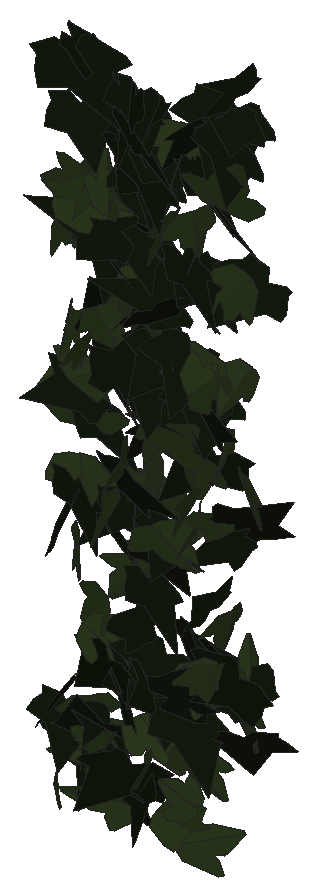
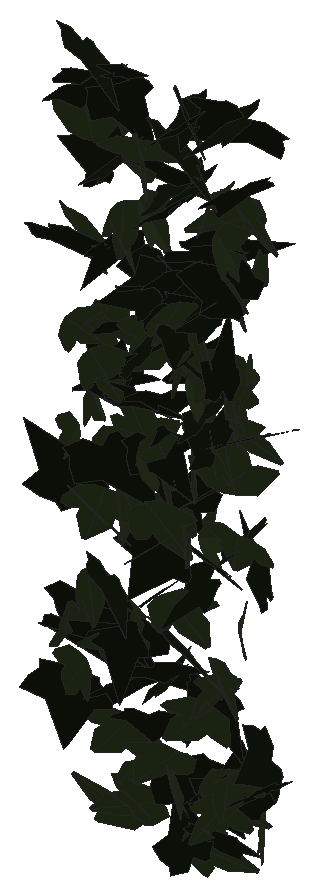
# SketchUp Ruby script. Lengths in inches.
U = 1.inch
M = Sketchup.active_model
def pt(a) = Geom::Point3d.new(a.map { |v| v * U })
def face(e, loops, mat)
  f = e.add_face(loops[0].map { |a| pt(a) })
  loops[1..].each { |l| e.add_face(l.map { |a| pt(a) }).erase! }
  f.material = f.back_material = mat if mat
  f
end
# faces: each face lists its corners as indices into pts; further lists are holes
def faces(e, pts, list, mat = nil) = list.each { |f| face(e, (f[0].is_a?(Array) ? f : [f]).map { |l| l.map { |i| pts[i] } }, mat) }
# xy, xz, yz: faces in a plane at the given z, y or x. An outline is a flat list of corners, or four numbers for a rectangle; further outlines are holes
def ring(l) = l.size == 4 ? [[l[0], l[1]], [l[2], l[1]], [l[2], l[3]], [l[0], l[3]]] : l.each_slice(2).to_a
def flat(e, list, mat, &to3) = list.each { |f| face(e, (f[0].is_a?(Array) ? f : [f]).map { |l| ring(l).map { |u, v| to3.(u, v) } }, mat) }
def xy(e, z, list, mat = nil) = flat(e, list, mat) { |x, y| [x, y, z] }
def xz(e, y, list, mat = nil) = flat(e, list, mat) { |x, z| [x, y, z] }
def yz(e, x, list, mat = nil) = flat(e, list, mat) { |y, z| [x, y, z] }
def lines(e, pts, list) = list.each { |a, b| e.add_line(pt(pts[a]), pt(pts[b])) }
# prism: a flat outline (further loops are holes) pulled along v
def prism(e, loops, v, mat = nil)
  f = face(e, loops, mat); d = Geom::Vector3d.new(v.map { |x| x * U })
  f.pushpull(f.normal.samedirection?(d) ? d.length : -d.length)
end
def box(e, o, s, mat = nil) = prism(e, [[o, [o[0] + s[0], o[1], o[2]], [o[0] + s[0], o[1] + s[1], o[2]], [o[0], o[1] + s[1], o[2]]]], [0, 0, s[2]], mat)
def at(x, y, z, deg = 0) = Geom::Transformation.translation(pt([x, y, z])) * Geom::Transformation.rotation(ORIGIN, Z_AXIS, deg.degrees)
def axes(o, x, y, z) = Geom::Transformation.new([*x, 0, *y, 0, *z, 0, *pt(o).to_a, 1])
def part(name) = M.definitions.add(name)
# library, detail: a bought-in or finely detailed component or shape, given as its bounding box
def library(name, o, s) = part(name).tap { |d| box(d.entities, o, s) }
def detail(e, o, s) = box(e.add_group.entities, o, s)
def put(e, d, t, mat = nil) = e.add_instance(d, t).tap { |i| i.material = mat if mat }
def group(e, t, mat = nil) = e.add_group.tap { |g| g.transformation = t; g.material = mat if mat }.entities
root = M.entities
M.materials.add("1026 AP 7946 SUNNY SIDE UP").color = [254, 231, 186]
M.materials.add("efeu1").color = [18, 25, 13]
M.materials.add("efeu2").color = [43, 57, 29]
c1 = part("ivyleaf_10")
p = [[0,0.5,-0.03],[-0.0625,2.02,-0.43],[-0.19,2.01,-0.46],[-0.54,1.05,-0.29],[-0.52,0.625,-0.18],[-0.83,0.76,-0.28],
  [-1.16,0.64,-0.33],[-1.15,0.33,-0.24],[-0.77,-0.39,0.02],[-0.3,-0.51,0.16],[0.04,-0.48,0.23],[-0.02,2.01,-0.4375],
  [-0.06,2.01,-0.43],[0.04,-0.49,0.23],[0.67,-0.49,0.14],[1.38,0.36,-0.2],[1.375,0.51,-0.24],[0.81,0.65,-0.19],
  [0.62,0.59,-0.15],[0.6,1.09,-0.28],[0.5,1.23,-0.31]]
faces(c1.entities,p,[[0,1,2,3,4,5,6,7,8,9,10],[11,12,0,13,14,15,16,17,18,19,20]],"efeu2")
c2 = part("ivyleaf_9")
p = [[1.54,2.16,1.25],[1.36,2.04,1.19],[-0.21,0.99,0.68],[-0.71,1.11,0.82],[-0.85,0.86,0.67],[-0.8,0.17,0.21],
  [-0.9,-0.01,0.1],[-0.67,-0.16,-0.02],[-0.08,-0.08,-0.05],[-0.03,-0.6,-0.4],[0.65,-0.88,-0.66],[0.83,-0.6,-0.49],
  [1.29,-0.42,-0.43],[1.8125,-0.07,-0.26],[1.21,0.44,0.15]]
faces(c2.entities,p,[[0,1,2,3,4,5,6,7,8,9,10,11,12,13,14]],"efeu1")
put(root,c1,axes([121.98,211.52,277.31],[0.03171,0.08334,0.32849],[0.20526,0.2908,-0.08524],[-0.47506,0.13121,-0.0149]),"1026 AP 7946 SUNNY SIDE UP")
put(root,c2,axes([121.49,211.78,272],[0.02452,0.24373,0.23934],[-0.06911,-0.22772,0.24931],[0.52342,-0.04148,0.02171]),"1026 AP 7946 SUNNY SIDE UP")
put(root,c2,axes([122.73,211.57,274.8125],[-0.20002,-0.06797,0.29588],[0.33643,0.19479,0.14606],[-0.32051,0.24688,-0.03133]),"1026 AP 7946 SUNNY SIDE UP")
put(root,c1,axes([122,211.64,277.5],[0.1599,-0.14005,-0.28907],[-0.3313,0.18686,-0.17415],[0.36373,0.23176,-0.03154]),"1026 AP 7946 SUNNY SIDE UP")
put(root,c2,axes([123.08,212.01,270.04],[-0.16156,-0.09203,0.26941],[-0.07925,-0.26858,-0.1191],[0.42945,-0.08418,0.07937]),"1026 AP 7946 SUNNY SIDE UP")
put(root,c2,axes([123.3,211.59,276.1],[0.17775,0.27835,0.04444],[0.04748,0.03253,-0.30889],[-0.43998,0.11597,-0.01538]),"1026 AP 7946 SUNNY SIDE UP")
put(root,c1,axes([122.26,212,272.6],[0.0991,-0.11712,0.28965],[0.16515,-0.26187,-0.13784],[0.45057,0.12174,-0.01318]),"1026 AP 7946 SUNNY SIDE UP")
put(root,c2,axes([122.66,211.8,278.65],[0.36741,-0.24284,-0.07309],[-0.09666,0.03725,-0.34646],[0.38526,0.24093,-0.01722]),"1026 AP 7946 SUNNY SIDE UP")
put(root,c1,axes([124.17,211.77,270.86],[-0.29442,-0.23757,-0.04002],[0.06154,0.0168,-0.31083],[0.37314,-0.19022,0.01968]),"1026 AP 7946 SUNNY SIDE UP")
put(root,c2,axes([124.53,211.8,270.88],[0.10748,0.01102,-0.34467],[-0.45516,-0.16967,-0.06767],[-0.26453,0.29641,-0.02361]),"1026 AP 7946 SUNNY SIDE UP")
put(root,c1,axes([122.68,211.65,273.58],[0.01249,-0.2277,-0.23311],[-0.01185,0.22486,-0.2334],[0.50319,0.01094,0.00029]),"1026 AP 7946 SUNNY SIDE UP")
put(root,c2,axes([122.7,211.86,268.9],[0.12076,0.13717,-0.30129],[-0.16617,-0.27424,-0.16228],[-0.48116,0.12914,-0.01957]),"1026 AP 7946 SUNNY SIDE UP")
put(root,c2,axes([123.58,211.89,276.83],[0.15184,-0.28554,-0.01731],[-0.01676,0.01242,-0.31039],[0.44931,0.09696,-0.00573]),"1026 AP 7946 SUNNY SIDE UP")
put(root,c1,axes([123.93,211.76,270.77],[-0.28756,-0.03559,-0.23541],[0.35968,0.01327,-0.19081],[0.05136,-0.29222,0.01827]),"1026 AP 7946 SUNNY SIDE UP")
put(root,c1,axes([124.01,211.5625,275.1875],[0.09265,0.02287,-0.32986],[0.16457,0.30652,0.04417],[0.47738,-0.1101,0.04879]),"1026 AP 7946 SUNNY SIDE UP")
put(root,c2,axes([122.39,211.97,276.82],[-0.26474,-0.19951,-0.20035],[-0.10805,-0.18914,0.26162],[-0.42328,0.17307,0.05853]),"1026 AP 7946 SUNNY SIDE UP")
put(root,c2,axes([123.64,211.95,269.94],[-0.06302,-0.3296,-0.06102],[0.04817,0.05391,-0.34088],[0.52385,-0.04461,0.02401]),"1026 AP 7946 SUNNY SIDE UP")
put(root,c2,axes([123.62,212.01,275.38],[-0.23731,-0.27407,0.02875],[-0.00163,-0.03303,-0.32215],[0.43343,-0.15018,0.01453]),"1026 AP 7946 SUNNY SIDE UP")
put(root,c1,axes([124.33,211.84,277.98],[-0.50833,-0.04495,0.06679],[0.09482,0.03719,0.33523],[-0.08049,0.32767,-0.0269]),"1026 AP 7946 SUNNY SIDE UP")
put(root,c1,axes([121.66,211.63,268.39],[-0.04245,0.09866,0.2925],[-0.294,0.21699,-0.09491],[-0.369,-0.18423,0.04197]),"1026 AP 7946 SUNNY SIDE UP")
put(root,c2,axes([123.52,211.72,270.28],[0.17481,0.0334,0.30119],[0.46174,0.00414,-0.11558],[-0.0248,0.31258,-0.0288]),"1026 AP 7946 SUNNY SIDE UP")
put(root,c2,axes([121.67,211.99,272.72],[0.10287,-0.2898,0.06343],[0.00913,-0.06347,-0.30632],[0.46631,0.06518,-0.008]),"1026 AP 7946 SUNNY SIDE UP")
put(root,c2,axes([121.87,212.06,274.18],[-0.32958,-0.06615,0.20746],[-0.17787,-0.20513,-0.19155],[0.28253,-0.20631,0.12141]),"1026 AP 7946 SUNNY SIDE UP")
put(root,c2,axes([122.43,212.07,269.72],[0.0155,-0.1148,0.25429],[0.0071,-0.24755,-0.11993],[0.42892,0.00824,-0.0072]),"1026 AP 7946 SUNNY SIDE UP")
put(root,c2,axes([122.65,212,278.86],[-0.27293,0.04592,-0.26828],[0.37081,-0.11474,-0.18326],[-0.18902,-0.2914,0.02787]),"1026 AP 7946 SUNNY SIDE UP")
put(root,c1,axes([121.57,212.04,275.2],[-0.02318,0.1366,-0.26729],[0.01022,-0.26034,-0.14269],[-0.46202,-0.01261,0.01025]),"1026 AP 7946 SUNNY SIDE UP")
put(root,c2,axes([122.8,212,268.62],[-0.2349,0.00883,-0.2457],[0.35356,-0.08929,-0.14899],[-0.12604,-0.26693,0.03998]),"1026 AP 7946 SUNNY SIDE UP")
put(root,c1,axes([123.25,211.82,272.63],[-0.3563,-0.15059,-0.16466],[0.24248,0.05267,-0.27754],[0.24445,-0.27174,0.03531]),"1026 AP 7946 SUNNY SIDE UP")
put(root,c2,axes([124.22,212.11,278.6875],[-0.0819,-0.29887,0.12323],[0.00144,-0.12303,-0.31254],[0.50719,-0.04791,0.02079]),"1026 AP 7946 SUNNY SIDE UP")
put(root,c1,axes([122.42,211.69,277.36],[0.03492,0.24385,-0.22842],[-0.04464,0.2242,0.25084],[0.51779,0.00288,0.03703]),"1026 AP 7946 SUNNY SIDE UP")
put(root,c1,axes([124.07,211.92,275.24],[-0.15284,0.02069,0.28333],[-0.41805,-0.08415,-0.09081],[0.11468,-0.27918,0.04658]),"1026 AP 7946 SUNNY SIDE UP")
put(root,c1,axes([123.58,211.99,268.58],[-0.01373,0.22535,0.17325],[-0.0109,-0.1671,0.23108],[0.44079,0.00289,0.01111]),"1026 AP 7946 SUNNY SIDE UP")
put(root,c2,axes([123.86,212.06,277.74],[0.24285,-0.20743,0.20604],[0.15007,-0.1787,-0.26633],[0.42887,0.17999,-0.02348]),"1026 AP 7946 SUNNY SIDE UP")
put(root,c1,axes([121.6,211.77,276.83],[0.0942,-0.26674,-0.21022],[0.11199,0.2112,-0.2636],[0.5146,0.00287,0.09585]),"1026 AP 7946 SUNNY SIDE UP")
put(root,c2,axes([123.72,212.09,274.47],[0.09045,-0.0918,0.30273],[0.16388,-0.27605,-0.11128],[0.45634,0.11733,-0.02004]),"1026 AP 7946 SUNNY SIDE UP")
put(root,c2,axes([122.39,212.04,273.01],[0.17115,-0.12462,0.27512],[0.26346,-0.20895,-0.17157],[0.38243,0.19971,-0.00493]),"1026 AP 7946 SUNNY SIDE UP")
put(root,c1,axes([123.64,212.03,273.23],[0.08484,-0.27749,0.09385],[0.00494,-0.09368,-0.29141],[0.45999,0.05218,-0.01418]),"1026 AP 7946 SUNNY SIDE UP")
put(root,c2,axes([122.89,212.04,271.67],[0.08663,-0.29451,-0.02554],[0.00072,0.0236,-0.30849],[0.46451,0.05489,0.00524]),"1026 AP 7946 SUNNY SIDE UP")
put(root,c2,axes([123.13,212.16,275.16],[-0.24788,-0.22455,0.11691],[-0.08986,-0.1,-0.28305],[0.38621,-0.16739,0.00918]),"1026 AP 7946 SUNNY SIDE UP")
put(root,c1,axes([121.85,212.03,274.42],[-0.28382,0.02903,0.23839],[-0.32949,-0.14822,-0.1502],[0.16038,-0.25314,0.11328]),"1026 AP 7946 SUNNY SIDE UP")
put(root,c2,axes([121.47,211.6875,269.41],[0.08976,0.14286,0.2929],[0.13574,0.27021,-0.1566],[-0.48037,0.10305,0.01048]),"1026 AP 7946 SUNNY SIDE UP")
put(root,c1,axes([122.1,212.1,268.96],[0.03566,-0.24912,0.15025],[0.04365,-0.14516,-0.25823],[0.45294,0.0336,0.01306]),"1026 AP 7946 SUNNY SIDE UP")
put(root,c1,axes([123.1875,212.08,277.2],[0.09765,-0.30046,0.10814],[0.02161,-0.10606,-0.3166],[0.50088,0.06315,-0.00742]),"1026 AP 7946 SUNNY SIDE UP")
put(root,c2,axes([122.46,212.23,277.74],[-0.10113,-0.17305,0.26027],[-0.00544,-0.2587,-0.18426],[0.48275,-0.03917,0.05244]),"1026 AP 7946 SUNNY SIDE UP")
put(root,c2,axes([123.82,212.01,278.87],[-0.06374,0.24318,-0.19961],[0.03519,-0.194,-0.25499],[-0.489,-0.04566,0.00767]),"1026 AP 7946 SUNNY SIDE UP")
put(root,c2,axes([122.26,211.9375,270.31],[0.19729,-0.00263,-0.29696],[-0.44595,-0.0573,-0.12698],[-0.08099,0.3091,-0.02419]),"1026 AP 7946 SUNNY SIDE UP")
put(root,c1,axes([123.27,212.03,273.8125],[-0.44047,-0.00411,0.1513],[0.23077,0.00799,0.28861],[-0.01156,0.3162,-0.00348]),"1026 AP 7946 SUNNY SIDE UP")
put(root,c1,axes([123.75,212.03,270.57],[0.32985,0.18,-0.03032],[-0.01527,-0.03532,-0.2842],[-0.28665,0.20901,-0.01975]),"1026 AP 7946 SUNNY SIDE UP")
put(root,c1,axes([124.41,212.04,276.64],[0.40483,-0.20682,-0.08454],[-0.12657,0.02852,-0.33887],[0.32544,0.26836,-0.02662]),"1026 AP 7946 SUNNY SIDE UP")
put(root,c1,axes([123.66,212,269.3125],[-0.39525,-0.00479,-0.13824],[0.21045,-0.0312,-0.25736],[-0.0165,-0.28322,0.02901]),"1026 AP 7946 SUNNY SIDE UP")
put(root,c2,axes([121.38,212.2,269.13],[-0.11273,-0.27337,0.05892],[-0.01362,-0.05845,-0.29141],[0.43945,-0.07194,0.00609]),"1026 AP 7946 SUNNY SIDE UP")
put(root,c1,axes([123.57,212,268.01],[0.27196,-0.06873,-0.26895],[0.41644,-0.01451,0.18489],[-0.07915,-0.3125,0.04864]),"1026 AP 7946 SUNNY SIDE UP")
put(root,c1,axes([124.32,212.21,275.1875],[-0.12181,-0.18223,0.22118],[0.05434,-0.22814,-0.18708],[0.44071,-0.02224,0.0842]),"1026 AP 7946 SUNNY SIDE UP")
put(root,c2,axes([123.32,212.12,275.94],[-0.28735,0.0862,0.23044],[-0.37593,-0.07656,-0.17166],[0.01442,-0.27812,0.11676]),"1026 AP 7946 SUNNY SIDE UP")
put(root,c1,axes([122.84,212.01,268.91],[0.1,-0.26874,-0.07806],[-0.02574,0.07242,-0.28407],[0.43764,0.06567,0.00113]),"1026 AP 7946 SUNNY SIDE UP")
put(root,c1,axes([121.79,212.02,274.92],[0.016,-0.30212,-0.06905],[0.01557,0.06563,-0.31079],[0.48577,0.00784,0.01224]),"1026 AP 7946 SUNNY SIDE UP")
put(root,c1,axes([124.14,212.12,274.18],[-0.1339,0.24627,-0.1302],[-0.10769,-0.14819,-0.24806],[-0.42276,-0.04025,0.10443]),"1026 AP 7946 SUNNY SIDE UP")
put(root,c2,axes([121.59,212.1,279.16],[-0.16337,-0.18074,-0.30345],[0.40386,0.16388,-0.19665],[0.3615,-0.26476,0.08256]),"1026 AP 7946 SUNNY SIDE UP")
put(root,c1,axes([123.31,211.96,268.26],[0.18336,0.0706,0.27185],[0.34872,0.1423,-0.13956],[-0.24972,0.25054,0.00472]),"1026 AP 7946 SUNNY SIDE UP")
put(root,c2,axes([122.7,212.25,277.67],[0.01316,-0.28013,0.13766],[0.04692,-0.13392,-0.28851],[0.48686,0.02048,0.02408]),"1026 AP 7946 SUNNY SIDE UP")
put(root,c2,axes([122.97,212.22,270.5],[-0.32511,-0.19697,0.02318],[-0.00277,-0.03229,-0.2935],[0.31192,-0.20559,0.02155]),"1026 AP 7946 SUNNY SIDE UP")
put(root,c1,axes([122.33,212.17,274.9],[0.08267,-0.27752,0.10449],[0.02336,-0.10201,-0.29155],[0.46487,0.05448,-0.00393]),"1026 AP 7946 SUNNY SIDE UP")
put(root,c2,axes([124.05,212.22,279.07],[-0.29665,-0.25465,-0.02007],[0.03291,0.00693,-0.32619],[0.40007,-0.18939,0.01195]),"1026 AP 7946 SUNNY SIDE UP")
put(root,c1,axes([122.03,212.12,268.82],[0.1969,-0.01285,-0.25045],[-0.38154,-0.02777,-0.12745],[-0.02965,0.27199,-0.02323]),"1026 AP 7946 SUNNY SIDE UP")
put(root,c2,axes([121.65,212.14,268.87],[0.35629,0.06751,0.15882],[-0.24275,-0.01793,0.24236],[0.10396,-0.27326,0.02163]),"1026 AP 7946 SUNNY SIDE UP")
put(root,c2,axes([121.98,212.3,269.09],[-0.13209,-0.22666,0.15785],[-0.07589,-0.14686,-0.24983],[0.4246,-0.09676,0.00445]),"1026 AP 7946 SUNNY SIDE UP")
put(root,c2,axes([122.98,211.99,272.18],[0.41278,0.07968,-0.05115],[-0.06227,-0.04118,-0.28145],[-0.13426,0.26406,-0.02673]),"1026 AP 7946 SUNNY SIDE UP")
put(root,c2,axes([122.54,212.26,278.77],[-0.02326,-0.30912,0.04247],[-0.00304,-0.04293,-0.31907],[0.49072,-0.01492,0.00004]),"1026 AP 7946 SUNNY SIDE UP")
put(root,c2,axes([122.375,212.31,269.95],[-0.11488,-0.08092,0.25868],[-0.10274,-0.24736,-0.10297],[0.40261,-0.08621,0.04754]),"1026 AP 7946 SUNNY SIDE UP")
put(root,c1,axes([121.76,212.11,273.7],[-0.47116,-0.13702,0.04522],[0.04575,0.04342,0.33854],[-0.22194,0.29983,-0.0262]),"1026 AP 7946 SUNNY SIDE UP")
put(root,c1,axes([122.99,212.1,275.41],[-0.47765,0.06073,-0.12702],[0.17906,-0.05776,-0.31778],[-0.12189,-0.32285,0.03094]),"1026 AP 7946 SUNNY SIDE UP")
put(root,c2,axes([123.01,212.32,272.3],[-0.12022,-0.22814,0.15044],[-0.02902,-0.14833,-0.24737],[0.42604,-0.07448,0.0256]),"1026 AP 7946 SUNNY SIDE UP")
put(root,c1,axes([122.98,212.06,273.43],[0.24745,-0.21552,-0.12584],[-0.06535,0.11824,-0.27213],[0.38305,0.1594,0.03487]),"1026 AP 7946 SUNNY SIDE UP")
put(root,c2,axes([122.81,212.26,274.67],[-0.24804,-0.23634,-0.05364],[0.08727,0.02355,-0.29066],[0.36994,-0.16402,0.0326]),"1026 AP 7946 SUNNY SIDE UP")
put(root,c1,axes([121.57,212.18,272.88],[0.45727,0.00263,0.09415],[0.14334,-0.03127,-0.29812],[0.01081,0.30322,-0.02976]),"1026 AP 7946 SUNNY SIDE UP")
put(root,c1,axes([122,212.08,275.36],[-0.29529,-0.20741,-0.11494],[0.16401,0.05305,-0.28515],[0.33105,-0.21129,0.03874]),"1026 AP 7946 SUNNY SIDE UP")
put(root,c2,axes([123.66,212.08,276.6],[0.06876,-0.21819,-0.21085],[-0.07858,0.19734,-0.22797],[0.46244,0.06598,-0.00739]),"1026 AP 7946 SUNNY SIDE UP")
put(root,c1,axes([123.66,212.01,272.79],[0.03582,-0.25261,-0.20585],[-0.03754,0.197,-0.2601],[0.50366,0.03265,-0.00474]),"1026 AP 7946 SUNNY SIDE UP")
put(root,c2,axes([123.84,212.21,274.36],[-0.36966,0.04454,0.1818],[-0.2839,-0.02405,-0.24203],[-0.03292,-0.29282,0.04577]),"1026 AP 7946 SUNNY SIDE UP")
put(root,c2,axes([124.52,212.12,270.48],[-0.42158,-0.12205,-0.06763],[-0.10215,-0.01391,0.30306],[-0.19192,0.27552,-0.01273]),"1026 AP 7946 SUNNY SIDE UP")
put(root,c2,axes([122.86,212.08,270.99],[-0.29053,0.21881,0.0941],[-0.12098,0.05255,-0.29371],[-0.35186,-0.19873,0.02329]),"1026 AP 7946 SUNNY SIDE UP")
put(root,c1,axes([122.27,212.17,268.07],[0.08903,0.00577,-0.2952],[-0.44867,0.02889,-0.05731],[0.04283,0.29068,0.01327]),"1026 AP 7946 SUNNY SIDE UP")
put(root,c2,axes([122.99,212.3,278.05],[-0.46332,-0.05695,0.04728],[-0.06079,-0.04198,-0.30749],[0.09801,-0.29529,0.03277]),"1026 AP 7946 SUNNY SIDE UP")
put(root,c2,axes([121.96,212.375,276.32],[-0.07183,-0.28673,0.10613],[-0.01085,-0.10481,-0.29958],[0.47982,-0.0453,0.00911]),"1026 AP 7946 SUNNY SIDE UP")
put(root,c2,axes([122.32,212.27,272.5625],[-0.4243,0.02142,-0.06995],[0.09855,-0.05578,-0.27456],[-0.05349,-0.27264,0.04901]),"1026 AP 7946 SUNNY SIDE UP")
put(root,c1,axes([121.39,212.36,271.625],[0.05236,-0.09061,0.28076],[0.29456,-0.20177,-0.0937],[0.34331,0.18695,0.03757]),"1026 AP 7946 SUNNY SIDE UP")
put(root,c1,axes([121.92,212.05,270.5625],[0.06034,0.22448,0.181],[0.06047,0.17029,-0.2335],[-0.44289,0.05383,-0.00722]),"1026 AP 7946 SUNNY SIDE UP")
put(root,c1,axes([123.55,212.17,273.67],[-0.44536,0.08088,0.03049],[-0.05506,-0.01693,-0.30239],[-0.12345,-0.28423,0.02488]),"1026 AP 7946 SUNNY SIDE UP")
put(root,c2,axes([123.61,212.34,274.66],[-0.18309,-0.27389,-0.04254],[0.04067,0.03215,-0.3062],[0.43328,-0.11876,0.01077]),"1026 AP 7946 SUNNY SIDE UP")
put(root,c2,axes([122.24,212.36,268.04],[0.4115,-0.13525,-0.11826],[0.18174,-0.02342,0.30175],[-0.21058,-0.2845,0.02933]),"1026 AP 7946 SUNNY SIDE UP")
put(root,c2,axes([121.74,212.34,275.2],[0.11188,0.15396,0.28336],[-0.21561,-0.23779,0.17282],[0.44496,-0.15393,0.01249]),"1026 AP 7946 SUNNY SIDE UP")
put(root,c2,axes([123.45,212.26,278.04],[0.24067,-0.27308,-0.06117],[-0.03511,0.05376,-0.32211],[0.43751,0.15453,0.0078]),"1026 AP 7946 SUNNY SIDE UP")
put(root,c1,axes([124.35,212.23,273.58],[-0.25878,0.21622,-0.08266],[0.06365,-0.07149,-0.28013],[-0.35769,-0.16915,0.00995]),"1026 AP 7946 SUNNY SIDE UP")
put(root,c2,axes([121.5,212.32,278.21],[-0.02052,-0.30272,-0.06773],[0.01578,0.06364,-0.31169],[0.48627,-0.01484,0.00725]),"1026 AP 7946 SUNNY SIDE UP")
put(root,c2,axes([121.94,212.27,276.25],[0.358,-0.21004,0.02264],[0.00317,-0.0319,-0.31849],[0.33225,0.22662,-0.02136]),"1026 AP 7946 SUNNY SIDE UP")
put(root,c1,axes([124.04,212.23,271.45],[-0.05243,-0.28635,-0.04126],[0.0211,0.0371,-0.29663],[0.4538,-0.03481,0.00902]),"1026 AP 7946 SUNNY SIDE UP")
put(root,c2,axes([122.79,212.1,278.46],[-0.2237,0.28351,0.07926],[-0.07284,0.06096,-0.32612],[-0.45548,-0.14899,0.01323]),"1026 AP 7946 SUNNY SIDE UP")
put(root,c1,axes([123.25,212.2,278.1875],[0.18472,-0.26947,-0.10006],[-0.02491,0.09705,-0.30134],[0.44889,0.11627,0.02445]),"1026 AP 7946 SUNNY SIDE UP")
put(root,c2,axes([122.45,212.32,276.67],[-0.01966,-0.29732,-0.08282],[0.0044,0.07866,-0.30611],[0.48359,-0.0128,-0.00059]),"1026 AP 7946 SUNNY SIDE UP")
put(root,c1,axes([122.57,212.32,271.63],[-0.28979,-0.16134,0.16716],[-0.1697,-0.12376,-0.25235],[0.31843,-0.21278,0.01765]),"1026 AP 7946 SUNNY SIDE UP")
put(root,c1,axes([123.5,212.33,276.9375],[0.22989,-0.26631,0.0607],[0.02896,-0.05878,-0.31308],[0.42841,0.14688,-0.01141]),"1026 AP 7946 SUNNY SIDE UP")
put(root,c2,axes([124.55,212.38,276.58],[-0.44371,-0.08867,0.0135],[-0.00765,-0.02973,-0.30363],[0.14085,-0.28095,0.02604]),"1026 AP 7946 SUNNY SIDE UP")
put(root,c1,axes([122.51,212.13,272.83],[0.2063,-0.17673,-0.18495],[-0.04368,0.18997,-0.21366],[0.39258,0.11401,0.07342]),"1026 AP 7946 SUNNY SIDE UP")
put(root,c2,axes([124.24,212.28,272.71],[-0.42487,0.12834,-0.02818],[0.02173,-0.0361,-0.30716],[-0.20543,-0.26925,0.02579]),"1026 AP 7946 SUNNY SIDE UP")
put(root,c2,axes([122.59,212.28,275.71],[-0.25237,0.22666,-0.15004],[0.11229,-0.12923,-0.28648],[-0.40962,-0.17507,0.01391]),"1026 AP 7946 SUNNY SIDE UP")
put(root,c2,axes([122.18,212.44,277.11],[-0.3331,-0.20614,0.04223],[-0.02175,-0.04606,-0.30385],[0.33013,-0.21103,0.0226]),"1026 AP 7946 SUNNY SIDE UP")
put(root,c1,axes([121.6875,212.29,276.74],[0.31188,-0.23087,-0.01863],[-0.02234,0.00991,-0.31347],[0.3633,0.19881,-0.00328]),"1026 AP 7946 SUNNY SIDE UP")
put(root,c2,axes([124.39,212.15,269.78],[0.2782,0.21877,-0.08798],[-0.06559,-0.07753,-0.28986],[-0.36413,0.18111,-0.015]),"1026 AP 7946 SUNNY SIDE UP")
put(root,c2,axes([121.96,212.43,274.68],[0.10999,-0.27554,0.11532],[0.03687,-0.11114,-0.29348],[0.46713,0.07365,-0.00399]),"1026 AP 7946 SUNNY SIDE UP")
put(root,c2,axes([121.79,212.45,274.32],[0.15538,-0.21756,0.20031],[0.10164,-0.18519,-0.24684],[0.44872,0.11728,-0.01345]),"1026 AP 7946 SUNNY SIDE UP")
put(root,c1,axes([122.8,212.32,273.89],[0.1208,0.25274,-0.11314],[-0.09181,-0.09801,-0.27147],[-0.4244,0.09314,0.02652]),"1026 AP 7946 SUNNY SIDE UP")
put(root,c1,axes([122.89,212.48,273.77],[0.07535,-0.14883,0.26262],[0.09146,-0.24931,-0.16213],[0.45623,0.07456,-0.01087]),"1026 AP 7946 SUNNY SIDE UP")
put(root,c2,axes([122.625,212.46,277.59],[-0.06382,-0.30048,0.06408],[-0.00572,-0.06399,-0.3127],[0.48301,-0.04046,0.00477]),"1026 AP 7946 SUNNY SIDE UP")
put(root,c2,axes([122.92,212.3,273.95],[-0.0273,0.21434,-0.19409],[0.00183,-0.18991,-0.22238],[-0.44998,-0.01378,0.01087]),"1026 AP 7946 SUNNY SIDE UP")
put(root,c1,axes([123.41,212.29,277.1875],[-0.12323,-0.29736,-0.02989],[0.10654,0.00981,-0.31007],[0.45729,-0.08242,0.06418]),"1026 AP 7946 SUNNY SIDE UP")
put(root,c1,axes([121.67,212.39,277.39],[0.03312,-0.29578,0.11132],[0.01135,-0.1095,-0.30612],[0.49594,0.02226,-0.00043]),"1026 AP 7946 SUNNY SIDE UP")
put(root,c2,axes([121.7,212.3,273.76],[0.1823,-0.25798,-0.09143],[0.01226,0.09797,-0.28706],[0.42806,0.10706,0.04716]),"1026 AP 7946 SUNNY SIDE UP")
put(root,c2,axes([123.04,212.52,275.18],[-0.0447,-0.16258,0.25311],[-0.00547,-0.24755,-0.16999],[0.46443,-0.01856,0.02236]),"1026 AP 7946 SUNNY SIDE UP")
put(root,c2,axes([121.48,212.23,279.24],[0.33392,-0.19704,-0.12669],[-0.06939,0.12788,-0.29149],[0.35762,0.2088,0.06174]),"1026 AP 7946 SUNNY SIDE UP")
put(root,c1,axes([124.18,212.3125,270.16],[-0.34694,0.16825,-0.09664],[0.08826,-0.0818,-0.28473],[-0.29053,-0.22577,0.02891]),"1026 AP 7946 SUNNY SIDE UP")
put(root,c2,axes([124.02,212.44,278.97],[-0.13023,-0.30387,-0.02645],[0.01507,0.02221,-0.32432],[0.47905,-0.0833,0.00301]),"1026 AP 7946 SUNNY SIDE UP")
put(root,c2,axes([122.07,212.23,272.14],[0.38847,-0.13142,-0.13167],[-0.16234,0.07597,-0.28732],[0.2372,0.26723,0.01899]),"1026 AP 7946 SUNNY SIDE UP")
put(root,c1,axes([121.67,212.3,269.31],[-0.26434,-0.20921,-0.04212],[0.06477,0.01767,-0.27555],[0.32851,-0.17183,0.02044]),"1026 AP 7946 SUNNY SIDE UP")
put(root,c1,axes([123.82,212.29,272.78],[-0.41311,-0.11206,-0.06165],[0.09843,0.00375,-0.29346],[0.17327,-0.26929,0.01972]),"1026 AP 7946 SUNNY SIDE UP")
put(root,c2,axes([124.15,212.3,272.86],[0.42552,0.13989,-0.02667],[0.01107,0.04408,0.31192],[0.22365,-0.26833,0.0353]),"1026 AP 7946 SUNNY SIDE UP")
put(root,c1,axes([122.51,212.34,276.05],[-0.16622,-0.27433,-0.05213],[0.23893,-0.01277,-0.2639],[0.36732,-0.11583,0.14807]),"1026 AP 7946 SUNNY SIDE UP")
put(root,c2,axes([124.21,212.15,279.39],[-0.12438,0.27953,0.1227],[-0.11007,0.10133,-0.29627],[-0.46391,-0.09899,0.0374]),"1026 AP 7946 SUNNY SIDE UP")
put(root,c1,axes([122.87,212.37,272.9],[-0.36133,-0.05773,0.19037],[-0.2524,-0.1044,-0.23943],[0.17106,-0.276,0.04884]),"1026 AP 7946 SUNNY SIDE UP")
put(root,c1,axes([123.1,212.36,278.33],[0.44248,0.11803,-0.0177],[-0.00923,-0.03196,-0.31331],[-0.18748,0.28015,-0.02634]),"1026 AP 7946 SUNNY SIDE UP")
put(root,c2,axes([122.86,212.375,276.31],[0.36179,-0.2058,0.04477],[0.032,-0.04406,-0.31767],[0.32958,0.23019,-0.0183]),"1026 AP 7946 SUNNY SIDE UP")
put(root,c1,axes([122.1,212.3,270.15],[-0.368,-0.06522,-0.16748],[0.26275,-0.00376,-0.24684],[0.08082,-0.28472,0.03987]),"1026 AP 7946 SUNNY SIDE UP")
put(root,c1,axes([121.85,212.28,270.89],[0.27101,-0.17507,-0.14934],[-0.1298,0.11996,-0.25139],[0.33193,0.18985,0.02363]),"1026 AP 7946 SUNNY SIDE UP")
put(root,c2,axes([123.81,212.14,271.52],[-0.07524,0.25899,0.14688],[-0.04482,0.13822,-0.2705],[-0.46158,-0.05564,0.00233]),"1026 AP 7946 SUNNY SIDE UP")
put(root,c2,axes([121.82,212.44,268.51],[-0.36762,-0.10518,-0.08448],[0.1368,0.00359,-0.26216],[0.15819,-0.24753,0.03039]),"1026 AP 7946 SUNNY SIDE UP")
put(root,c1,axes([122.69,212.26,269.3],[0.28949,0.19097,0.15791],[0.19695,0.08977,-0.27161],[-0.32962,0.22136,-0.0236]),"1026 AP 7946 SUNNY SIDE UP")
put(root,c2,axes([122.875,212.45,269.93],[-0.25632,-0.21229,-0.09086],[0.11839,0.05131,-0.27402],[0.34077,-0.17751,0.02685]),"1026 AP 7946 SUNNY SIDE UP")
put(root,c2,axes([123.65,212.42,273.64],[0.09241,0.1402,-0.29167],[-0.12265,-0.27346,-0.15734],[-0.48255,0.09635,-0.01587]),"1026 AP 7946 SUNNY SIDE UP")
put(root,c2,axes([123.52,212.25,270.92],[0.34483,-0.00538,-0.24272],[-0.37029,-0.01648,-0.22555],[-0.01321,0.32143,-0.01375]),"1026 AP 7946 SUNNY SIDE UP")
put(root,c1,axes([122.125,212.33,275.72],[-0.30935,0.21592,0.05395],[-0.19076,-0.04744,-0.27473],[-0.29213,-0.19766,0.12227]),"1026 AP 7946 SUNNY SIDE UP")
put(root,c1,axes([124.39,212.23,270.59],[0.05163,0.27204,-0.11546],[0.01677,0.11315,0.28294],[0.46326,-0.03441,0.00262]),"1026 AP 7946 SUNNY SIDE UP")
put(root,c1,axes([123.74,212.45,274.9375],[-0.15631,-0.25716,0.11066],[-0.04636,-0.10526,-0.28447],[0.43665,-0.10323,0.00941]),"1026 AP 7946 SUNNY SIDE UP")
put(root,c1,axes([122.4,212.3,275.41],[-0.1413,0.29638,0.02074],[-0.02098,0.01523,-0.31885],[-0.46645,-0.09046,0.00806]),"1026 AP 7946 SUNNY SIDE UP")
put(root,c1,axes([121.75,212.47,274.27],[0.27711,-0.18476,0.14868],[0.17966,-0.09146,-0.26299],[0.32306,0.20934,0.01873]),"1026 AP 7946 SUNNY SIDE UP")
put(root,c1,axes([121.76,212.26,268.88],[-0.21097,-0.21312,-0.19096],[0.21789,0.12764,-0.25544],[0.38557,-0.18874,0.03986]),"1026 AP 7946 SUNNY SIDE UP")
put(root,c2,axes([121.44,212.42,276.6875],[0.1968,-0.1267,0.25921],[0.36101,-0.115,-0.17747],[0.25844,0.25713,0.05053]),"1026 AP 7946 SUNNY SIDE UP")
